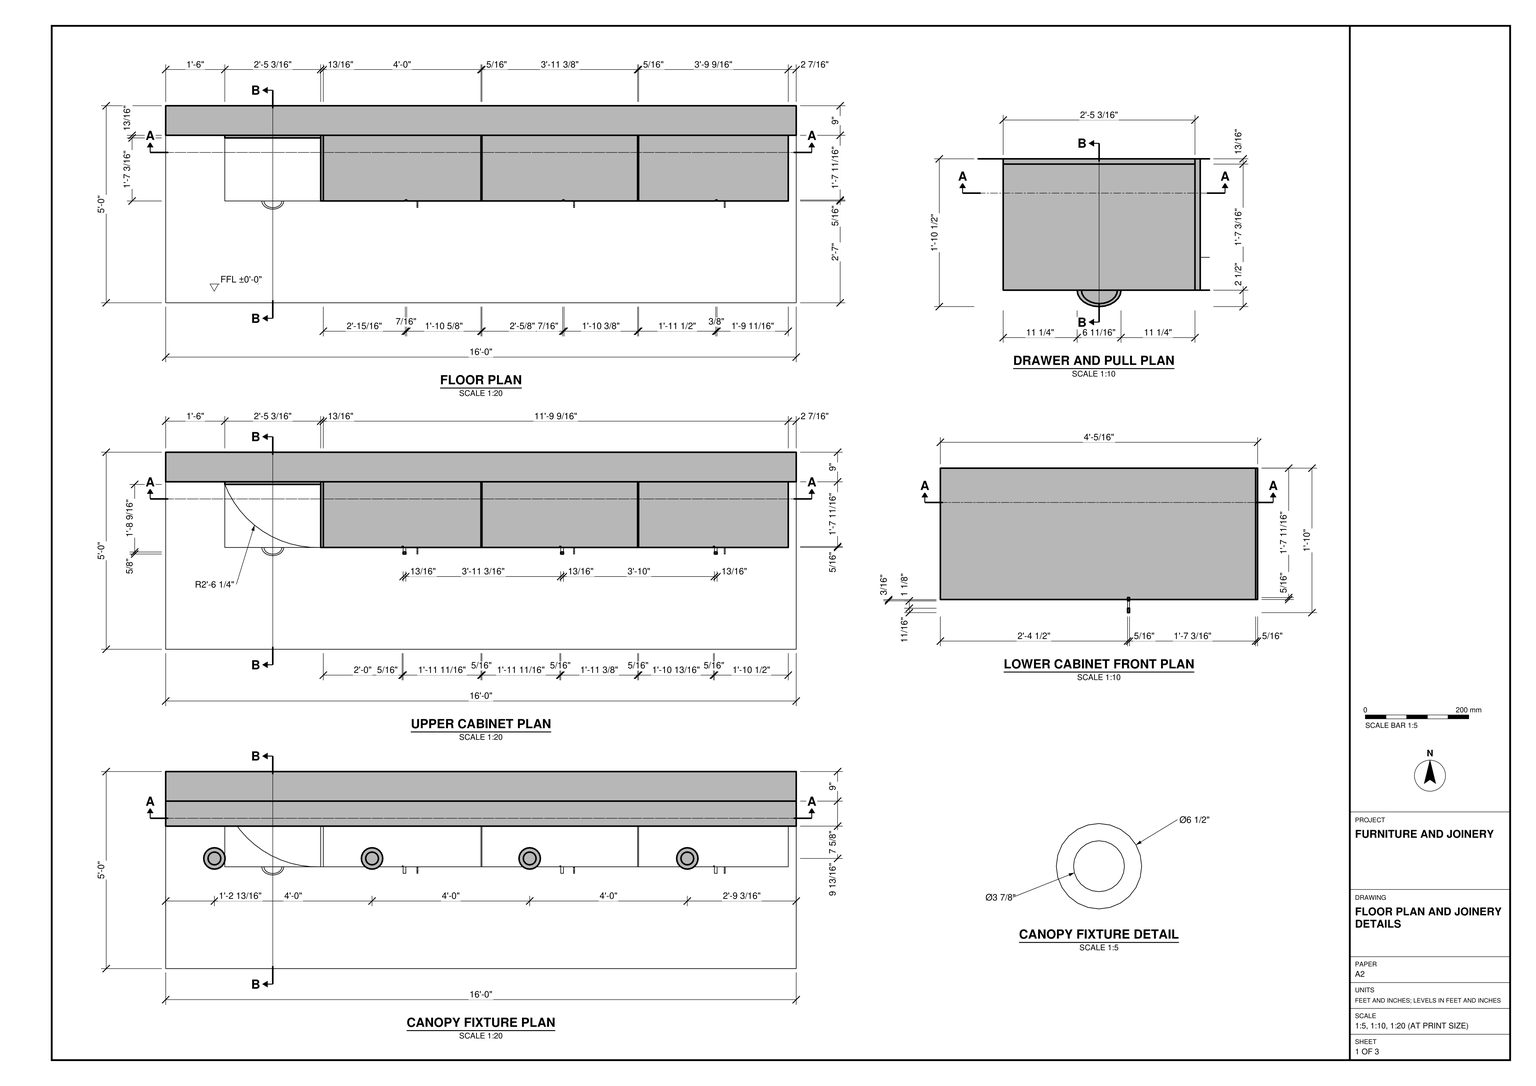
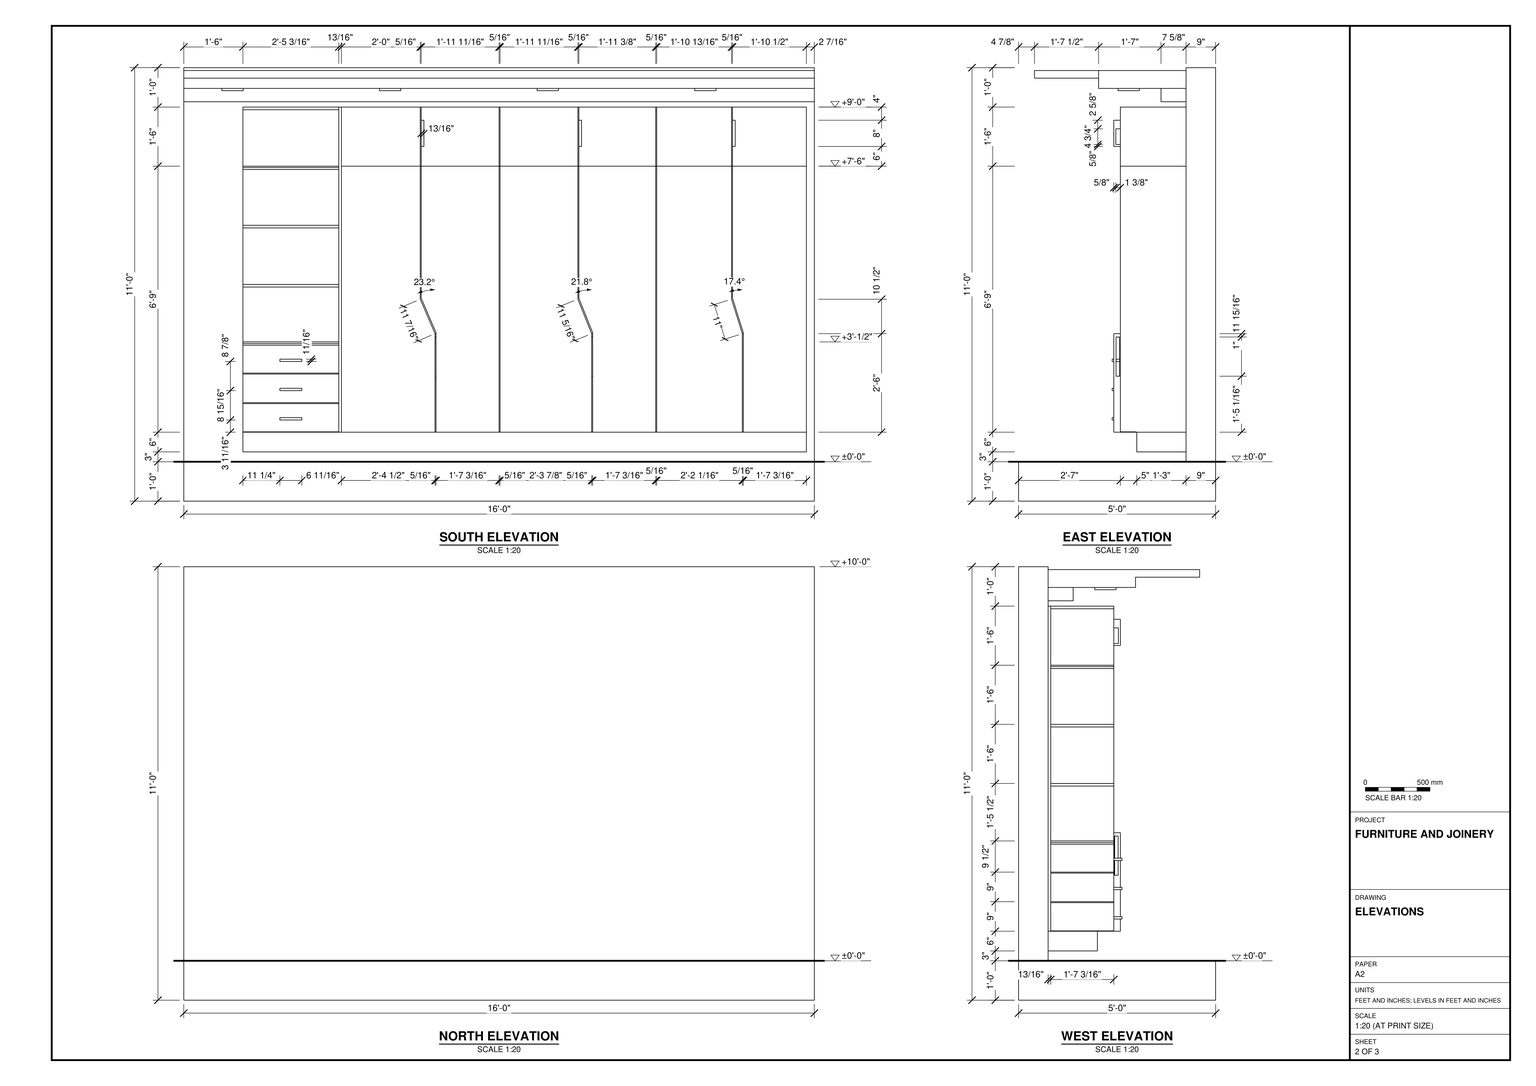
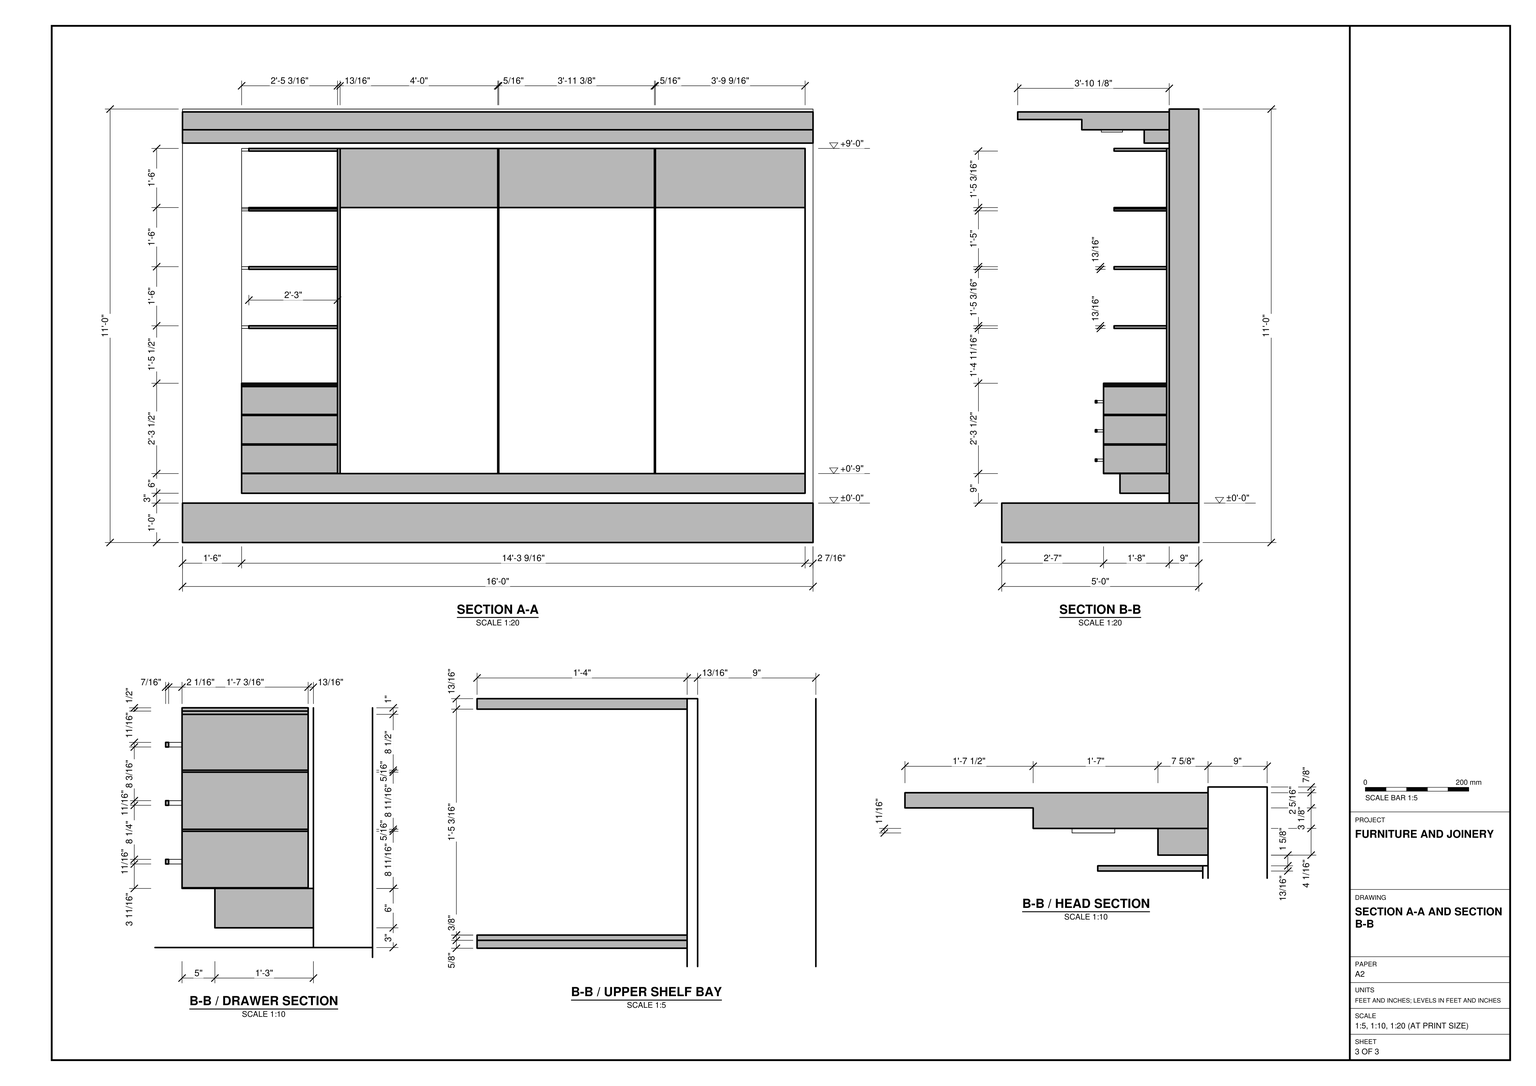
Build the storage wall in SketchUp from task_files/diagram_01.pdf. Work in feet and inches. The complete assembly is 16'-0" wide, 5'-0" deep and 11'-0" high. Use the top of the floor slab as the finished floor level, ±0'-0". The slab extends 1'-0" below this level, and the rear wall rises to +10'-0".

Use the south elevation to lay out the cabinet fronts. Leave 1'-6" between the left end of the wall and the narrow drawer and shelf bay. Model the three drawers with projecting pulls, the open shelves above them and the three wider cabinet bays to their right. Divide the wider bays into tall lower doors and a shorter row of upper doors. Follow the elevations for the door divisions and pull locations. Use the sections to set the shelf depths, panel thicknesses and recessed plinth rather than making the cabinet run a single solid block.

Above the cabinets, model the full-width projecting canopy with the stepped underside shown in the head section. Locate its fixtures from the canopy plan. Any decor or loose items shown may be represented by suitable library components. Keep the slab, rear wall, canopy and individual joinery pieces in separate groups or components, and use components for repeated parts. Save one SketchUp model as output_files/built_in_storage_wall_with_drawers_shelves_and_canopy.skp.

# SketchUp Ruby script. Lengths in inches.
U = 1.inch
M = Sketchup.active_model
def pt(a) = Geom::Point3d.new(a.map { |v| v * U })
def face(e, loops, mat)
  f = e.add_face(loops[0].map { |a| pt(a) })
  loops[1..].each { |l| e.add_face(l.map { |a| pt(a) }).erase! }
  f.material = f.back_material = mat if mat
  f
end
# faces: each face lists its corners as indices into pts; further lists are holes
def faces(e, pts, list, mat = nil) = list.each { |f| face(e, (f[0].is_a?(Array) ? f : [f]).map { |l| l.map { |i| pts[i] } }, mat) }
# xy, xz, yz: faces in a plane at the given z, y or x. An outline is a flat list of corners, or four numbers for a rectangle; further outlines are holes
def ring(l) = l.size == 4 ? [[l[0], l[1]], [l[2], l[1]], [l[2], l[3]], [l[0], l[3]]] : l.each_slice(2).to_a
def flat(e, list, mat, &to3) = list.each { |f| face(e, (f[0].is_a?(Array) ? f : [f]).map { |l| ring(l).map { |u, v| to3.(u, v) } }, mat) }
def xy(e, z, list, mat = nil) = flat(e, list, mat) { |x, y| [x, y, z] }
def xz(e, y, list, mat = nil) = flat(e, list, mat) { |x, z| [x, y, z] }
def yz(e, x, list, mat = nil) = flat(e, list, mat) { |y, z| [x, y, z] }
def lines(e, pts, list) = list.each { |a, b| e.add_line(pt(pts[a]), pt(pts[b])) }
# prism: a flat outline (further loops are holes) pulled along v
def prism(e, loops, v, mat = nil)
  f = face(e, loops, mat); d = Geom::Vector3d.new(v.map { |x| x * U })
  f.pushpull(f.normal.samedirection?(d) ? d.length : -d.length)
end
def box(e, o, s, mat = nil) = prism(e, [[o, [o[0] + s[0], o[1], o[2]], [o[0] + s[0], o[1] + s[1], o[2]], [o[0], o[1] + s[1], o[2]]]], [0, 0, s[2]], mat)
def at(x, y, z, deg = 0) = Geom::Transformation.translation(pt([x, y, z])) * Geom::Transformation.rotation(ORIGIN, Z_AXIS, deg.degrees)
def axes(o, x, y, z) = Geom::Transformation.new([*x, 0, *y, 0, *z, 0, *pt(o).to_a, 1])
def part(name) = M.definitions.add(name)
# library, detail: a bought-in or finely detailed component or shape, given as its bounding box
def library(name, o, s) = part(name).tap { |d| box(d.entities, o, s) }
def detail(e, o, s) = box(e.add_group.entities, o, s)
def put(e, d, t, mat = nil) = e.add_instance(d, t).tap { |i| i.material = mat if mat }
def group(e, t, mat = nil) = e.add_group.tap { |g| g.transformation = t; g.material = mat if mat }.entities
root = M.entities
M.materials.add("[Color D01]").color = [255, 242, 204]
M.materials.add("[Color M00]").color = [255, 255, 255]
M.materials.add("[Color M06]").color = [86, 86, 86]
M.materials.add("[Color M09]").color = [0, 0, 0]
M.materials.add("[Field Rectangle Tile]").color = [196, 189, 179]
M.materials.add("[Metal Corrugated Shiny]").color = [193, 193, 193]
M.materials.add("[Metal Rusted]").color = [184, 117, 91]
c1 = part("Group\#18")
prism(c1.entities,[[[0,1.91,0],[0.375,1.91,0],[0.43,1.5,0],[0.58,1.125,0],[0.83,0.8,0],[1.15,0.55,0],[1.53,0.4,0],[1.9375,0.34,0],[2.34,0.4,0],[2.72,0.55,0],[3.04,0.8,0],[3.29,1.125,0],[3.45,1.5,0],[3.5,1.91,0],[3.8125,1.91,0],[3.75,1.41,0],[3.56,0.95,0],[3.25,0.56,0],[2.86,0.26,0],[2.4,0.06,0],[1.91,0,0],[1.41,0.06,0],[0.95,0.26,0],[0.56,0.56,0],[0.26,0.95,0],[0.06,1.41,0]]],[0,0,0.5])
g1 = group(root,at(0,0,0))
xy(g1,0,[[0,0,192,60]])
xy(g1,12,[[0,0,192,60]],"[Field Rectangle Tile]")
xz(g1,0,[[0,0,192,12]])
xz(g1,60,[[0,0,192,12]])
yz(g1,0,[[0,0,60,12]])
yz(g1,192,[[0,0,60,12]])
g2 = group(root,at(0,51,12),"[Color D01]")
box(g2,[0,0,0],[192,9,120])
g3 = group(root,at(18,51,15),"[Color M06]")
g4 = group(g3,at(0,-15,0))
box(g4,[0,0,0],[171.58,15,6])
g5 = group(root,at(47.2,31,21),"[Color M06]")
box(g5,[0,0,0],[0.8,20,99])
g6 = group(root,at(48,31,21),"[Color M06]")
g7 = group(g6,at(0,0,81))
xy(g7,0,[[0,0,0,20,48,20,48,0,24.3,0,24.3,0.3,24,0.3,24,0],[48,0,48.3,20],[48.3,0,48.3,20,95.7,20,95.7,0,72.3,0,72.3,0.3,72,0.3,72,0],[95.7,0,96,20],[96,0,96,20,141.57,20,141.57,0,119.09,0,119.09,0.3,118.79,0.3,118.79,0]])
xy(g7,18,[[0,0,24,0,24,0.3,24.3,0.3,24.3,0,48,0,48,20,0,20],[48,0,48.3,20],[48.3,0,72,0,72,0.3,72.3,0.3,72.3,0,95.7,0,95.7,20,48.3,20],[95.7,0,96,20],[96,0,118.79,0,118.79,0.3,119.09,0.3,119.09,0,141.57,0,141.57,20,96,20]])
xz(g7,0,[[0,0,24,18],[24.3,0,48,18],[48,0,48.3,18],[48.3,0,72,18],[72.3,0,95.7,18],
  [95.7,0,96,18],[96,0,118.79,18],[119.09,0,141.57,18]])
xz(g7,0.3,[[24,0,24.3,18],[72,0,72.3,18],[118.79,0,119.09,18]])
xz(g7,20,[[0,0,48,18],[48,0,48.3,18],[48.3,0,95.7,18],[95.7,0,96,18],[96,0,141.57,18]])
yz(g7,0,[[0,0,20,18]])
yz(g7,24,[[0,0,0.3,18]])
yz(g7,24.3,[[0,0,0.3,18]])
yz(g7,48,[[0,0,20,18]])
yz(g7,48.3,[[0,0,20,18]])
yz(g7,72,[[0,0,0.3,18]])
yz(g7,72.3,[[0,0,0.3,18]])
yz(g7,95.7,[[0,0,20,18]])
yz(g7,96,[[0,0,20,18]])
yz(g7,118.79,[[0,0,0.3,18]])
yz(g7,119.09,[[0,0,0.3,18]])
yz(g7,141.57,[[0,0,20,18]])
g8 = group(g6,at(0,20,0))
g9 = group(g8,at(0,-20,0))
xy(g9,0,[[0,0,0,20,48,20,48,0,28.8,0,28.8,0.3,28.5,0.3,28.5,0],[48,0,48.3,20],[48.3,0,48.3,20,95.7,20,95.7,0,76.5,0,76.5,0.3,76.2,0.3,76.2,0],[95.7,0,96,20],[96,0,96,20,141.57,20,141.57,0,122.375,0,122.375,0.3,122.07,0.3,122.07,0]])
xy(g9,81,[[0,0,24,0,24,0.3,24.3,0.3,24.3,0,48,0,48,20,0,20],[48,0,48.3,20],[48.3,0,72,0,72,0.3,72.3,0.3,72.3,0,95.7,0,95.7,20,48.3,20],[95.7,0,96,20],[96,0,118.79,0,118.79,0.3,119.09,0.3,119.09,0,141.57,0,141.57,20,96,20]])
xz(g9,0,[[0,0,28.5,0,28.5,30,24,40.5,24,81,0,81],[28.8,0,48,0,48,81,24.3,81,24.3,40.8,28.8,30.3],[48,0,48.3,81],[48.3,0,76.2,0,76.2,30,72,40.5,72,81,48.3,81],[76.5,0,95.7,0,95.7,81,72.3,81,72.3,40.8,76.5,30.3],
  [95.7,0,96,81],[96,0,122.07,0,122.07,30,118.79,40.5,118.79,81,96,81],[122.375,0,141.57,0,141.57,81,119.09,81,119.09,40.8,122.375,30.3]])
xz(g9,0.3,[[28.5,0,28.8,0,28.8,30.3,24.3,40.8,24.3,81,24,81,24,40.5,28.5,30],[76.2,0,76.5,0,76.5,30.3,72.3,40.8,72.3,81,72,81,72,40.5,76.2,30],[122.07,0,122.375,0,122.375,30.3,119.09,40.8,119.09,81,118.79,81,118.79,40.5,122.07,30]])
xz(g9,20,[[0,0,48,81],[48,0,48.3,81],[48.3,0,95.7,81],[95.7,0,96,81],[96,0,141.57,81]])
yz(g9,0,[[0,0,20,81]])
yz(g9,24,[[0,40.5,0.3,81]])
yz(g9,24.3,[[0,40.8,0.3,81]])
yz(g9,28.5,[[0,0,0.3,30]])
yz(g9,28.8,[[0,0,0.3,30.3]])
yz(g9,48,[[0,0,20,81]])
yz(g9,48.3,[[0,0,20,81]])
yz(g9,72,[[0,40.5,0.3,81]])
yz(g9,72.3,[[0,40.8,0.3,81]])
yz(g9,76.2,[[0,0,0.3,30]])
yz(g9,76.5,[[0,0,0.3,30.3]])
yz(g9,95.7,[[0,0,20,81]])
yz(g9,96,[[0,0,20,81]])
yz(g9,118.79,[[0,40.5,0.3,81]])
yz(g9,119.09,[[0,40.8,0.3,81]])
yz(g9,122.07,[[0,0,0.3,30]])
yz(g9,122.375,[[0,0,0.3,30.3]])
yz(g9,141.57,[[0,0,20,81]])
p = [[24,0,40.5],[28.5,0,30],[28.5,0.3,30],[24,0.3,40.5],[72,0,40.5],[76.2,0,30],
  [76.2,0.3,30],[72,0.3,40.5],[118.79,0,40.5],[122.07,0,30],[122.07,0.3,30],[118.79,0.3,40.5],
  [28.8,0,30.3],[24.3,0,40.8],[24.3,0.3,40.8],[28.8,0.3,30.3],[76.5,0,30.3],[72.3,0,40.8],
  [72.3,0.3,40.8],[76.5,0.3,30.3],[122.375,0,30.3],[119.09,0,40.8],[119.09,0.3,40.8],[122.375,0.3,30.3]]
faces(g9,p,[[0,1,2,3],[4,5,6,7],[8,9,10,11],[12,13,14,15],[16,17,18,19],[20,21,22,23]])
g10 = group(root,at(76.5,29,21),"[Color M09]")
prism(g10,[[[0,2,30],[0,2,0],[0,0,0],[0,0,30]],[[0,1.8,28.99],[0,0.68,28.99],[0,0.68,17.05],[0,1.8,17.05]]],[0.3,0,0])
g11 = group(root,at(124.2,29,21),"[Color M09]")
prism(g11,[[[0,2,30],[0,2,0],[0,0,0],[0,0,30]],[[0,1.8,28.99],[0,0.68,28.99],[0,0.68,17.05],[0,1.8,17.05]]],[0.3,0,0])
g12 = group(root,at(170.08,29,21),"[Color M09]")
prism(g12,[[[0,2,30],[0,2,0],[0,0,0],[0,0,30]],[[0,1.74,28.99],[0,0.68,28.99],[0,0.68,17.05],[0,1.74,17.05]]],[0.3,0,0])
g13 = group(root,at(18,50.2,21),"[Color M06]")
box(g13,[0,0,0],[29.2,0.8,99])
g14 = group(root,at(18,31,119.7),"[Color M06]")
prism(g14,[[[29.2,19.2,-0.5],[29.2,0,-0.5],[26.1,0.05,-0.5],[23.01,0.42,-0.5],[19.99,1.1,-0.5],[17.05,2.1,-0.5],[14.22,3.38,-0.5],[11.54,4.95,-0.5],[9.04,6.79,-0.5],[6.74,8.87,-0.5],[4.67,11.18,-0.5],[2.84,13.6875,-0.5],[1.28,16.37,-0.5],[0,19.2,-0.5]]],[0,0,0.8])
g15 = group(root,at(18,31,101.6),"[Color M06]")
prism(g15,[[[29.2,19.2,0],[29.2,0,0],[26.1,0.05,0],[23.01,0.42,0],[19.99,1.1,0],[17.05,2.1,0],[14.22,3.38,0],[11.54,4.95,0],[9.04,6.79,0],[6.74,8.87,0],[4.67,11.18,0],[2.84,13.6875,0],[1.28,16.37,0],[0,19.2,0]]],[0,0,0.4])
g16 = group(root,at(18,31,83.7),"[Color M06]")
prism(g16,[[[29.2,19.2,-0.5],[29.2,0,-0.5],[26.1,0.05,-0.5],[23.01,0.42,-0.5],[19.99,1.1,-0.5],[17.05,2.1,-0.5],[14.22,3.38,-0.5],[11.54,4.95,-0.5],[9.04,6.79,-0.5],[6.74,8.87,-0.5],[4.67,11.18,-0.5],[2.84,13.6875,-0.5],[1.28,16.37,-0.5],[0,19.2,-0.5]]],[0,0,0.8])
g17 = group(root,at(18,31,65.7),"[Color M06]")
prism(g17,[[[29.2,19.2,-0.5],[29.2,0,-0.5],[26.1,0.05,-0.5],[23.01,0.42,-0.5],[19.99,1.1,-0.5],[17.05,2.1,-0.5],[14.22,3.38,-0.5],[11.54,4.95,-0.5],[9.04,6.79,-0.5],[6.74,8.87,-0.5],[4.67,11.18,-0.5],[2.84,13.6875,-0.5],[1.28,16.37,-0.5],[0,19.2,-0.5]]],[0,0,0.8])
g18 = group(root,at(18,31,101.3),"[Color M06]")
prism(g18,[[[29.2,19.2,-0.3],[29.2,0,-0.3],[26.1,0.05,-0.3],[23.01,0.42,-0.3],[19.99,1.1,-0.3],[17.05,2.1,-0.3],[14.22,3.38,-0.3],[11.54,4.95,-0.3],[9.04,6.79,-0.3],[6.74,8.87,-0.3],[4.67,11.18,-0.3],[2.84,13.6875,-0.3],[1.28,16.37,-0.3],[0,19.2,-0.3]]],[0,0,0.6])
g19 = group(root,at(18,31,21),"[Color M06]")
xy(g19,0,[[0,0,29.2,19.2]])
xy(g19,0.1,[[0,0,29.2,19.2]])
xy(g19,8.7,[[0,0,29.2,19.2]])
xy(g19,9,[[0,0,29.2,19.2]])
xy(g19,17.7,[[0,0,29.2,19.2]])
xy(g19,18,[[0,0,29.2,19.2]])
xy(g19,26.5,[[0,0,29.2,19.2]])
xy(g19,27,[[0,0,29.2,19.2]])
xy(g19,27.5,[[0,0,29.2,19.2]])
xz(g19,0,[[0,0,29.2,0.1],[0,0.1,29.2,8.7],[0,8.7,29.2,9],[0,9,29.2,17.7],[0,17.7,29.2,18],
  [0,18,29.2,26.5],[0,26.5,29.2,27],[0,27,29.2,27.5]])
xz(g19,19.2,[[0,0,29.2,0.1],[0,0.1,29.2,8.7],[0,8.7,29.2,9],[0,9,29.2,17.7],[0,17.7,29.2,18],
  [0,18,29.2,26.5],[0,26.5,29.2,27],[0,27,29.2,27.5]])
yz(g19,0,[[0,0,19.2,0.1],[0,0.1,19.2,8.7],[0,8.7,19.2,9],[0,9,19.2,17.7],[0,17.7,19.2,18],
  [0,18,19.2,26.5],[0,26.5,19.2,27],[0,27,19.2,27.5]])
yz(g19,29.2,[[0,0,19.2,0.1],[0,0.1,19.2,8.7],[0,8.7,19.2,9],[0,9,19.2,17.7],[0,17.7,19.2,18],
  [0,18,19.2,26.5],[0,26.5,19.2,27],[0,27,19.2,27.5]])
put(root,c1,axes([29.26,28.5,42.53],[1.75218,0,0],[0,1.31,0],[0,0,1.41]),"[Color M09]")
put(root,c1,axes([29.26,28.5,33.66],[1.75218,0,0],[0,1.31,0],[0,0,1.41]),"[Color M09]")
put(root,c1,axes([29.26,28.5,24.72],[1.75218,0,0],[0,1.31,0],[0,0,1.41]),"[Color M09]")
g20 = group(root,at(72.3,29,108),"[Color M09]")
prism(g20,[[[0.82,2,5.38],[0.82,2,8],[0.82,0,8],[0.82,0,0],[0.82,2,0],[0.82,2,0.62],[0.82,0.62,0.62],[0.82,0.62,5.38]]],[-0.82,0,0])
g21 = group(root,at(120.3,29,108),"[Color M09]")
prism(g21,[[[0.82,2,5.38],[0.82,2,8],[0.82,0,8],[0.82,0,0],[0.82,2,0],[0.82,2,0.62],[0.82,0.62,0.62],[0.82,0.62,5.38]]],[-0.82,0,0])
g22 = group(root,at(167.09,29,108),"[Color M09]")
prism(g22,[[[0.82,2,5.38],[0.82,2,8],[0.82,0,8],[0.82,0,0],[0.82,2,0],[0.82,2,0.62],[0.82,0.62,0.62],[0.82,0.62,5.38]]],[-0.82,0,0])
g23 = group(root,at(0,46,122),"[Color D01]")
xy(g23,-0.375,[[0,-2.625,192,5]])
xy(g23,3.6875,[[0,-2.625,192,5]],"[Color D01]")
xz(g23,-2.625,[[0,-0.375,192,3.6875]],"[Color D01]")
xz(g23,5,[[0,-0.375,192,3.6875]])
yz(g23,0,[[-2.625,-0.375,5,3.6875]])
yz(g23,192,[[-2.625,-0.375,5,3.6875]])
g24 = group(root,at(0,4.85,125.6875),"[Color M00]")
xy(g24,0,[[0,19.52,192,46.15]])
xy(g24,3.125,[[0,0,192,19.52]])
xy(g24,5.4375,[[0,0,192,46.15]])
xz(g24,0,[[0,3.125,192,5.4375]])
xz(g24,19.52,[[0,0,192,3.125]])
xz(g24,46.15,[[0,0,192,5.4375]])
yz(g24,0,[[19.52,0,19.52,3.125,0,3.125,0,5.4375,46.15,5.4375,46.15,0]])
yz(g24,192,[[19.52,0,46.15,5.4375],[0,3.125,19.52,5.4375]])
g25 = group(root,at(11.59,30.3,125),"[Metal Rusted]")
xy(g25,0,[[[3.25,0,2.41,0.11,1.625,0.44,0.95,0.95,0.44,1.625,0.11,2.41,0,3.25,0.11,4.09,0.44,4.875,0.95,5.55,1.625,6.06,2.41,6.39,3.25,6.5,4.09,6.39,4.875,6.06,5.55,5.55,6.06,4.875,6.39,4.09,6.5,3.25,6.39,2.41,6.06,1.625,5.55,0.95,4.875,0.44,4.09,0.11],[3.25,1.3125,3.75,1.38,4.22,1.57,4.62,1.88,4.93,2.28,5.12,2.75,5.1875,3.25,5.12,3.75,4.93,4.22,4.62,4.62,4.22,4.93,3.75,5.12,3.25,5.1875,2.75,5.12,2.28,4.93,1.88,4.62,1.57,4.22,1.38,3.75,1.3125,3.25,1.38,2.75,1.57,2.28,1.88,1.88,2.28,1.57,2.75,1.38]]])
xy(g25,0.4375,[[3.25,1.3125,3.75,1.38,4.22,1.57,4.62,1.88,4.93,2.28,5.12,2.75,5.1875,3.25,5.12,3.75,4.93,4.22,4.62,4.62,4.22,4.93,3.75,5.12,3.25,5.1875,2.75,5.12,2.28,4.93,1.88,4.62,1.57,4.22,1.38,3.75,1.3125,3.25,1.38,2.75,1.57,2.28,1.88,1.88,2.28,1.57,2.75,1.38]],"[Metal Corrugated Shiny]")
xy(g25,0.6875,[[[3.25,0,4.09,0.11,4.875,0.44,5.55,0.95,6.06,1.625,6.39,2.41,6.5,3.25,6.39,4.09,6.06,4.875,5.55,5.55,4.875,6.06,4.09,6.39,3.25,6.5,2.41,6.39,1.625,6.06,0.95,5.55,0.44,4.875,0.11,4.09,0,3.25,0.11,2.41,0.44,1.625,0.95,0.95,1.625,0.44,2.41,0.11],[3.25,1.3125,2.75,1.38,2.28,1.57,1.88,1.88,1.57,2.28,1.38,2.75,1.3125,3.25,1.38,3.75,1.57,4.22,1.88,4.62,2.28,4.93,2.75,5.12,3.25,5.1875,3.75,5.12,4.22,4.93,4.62,4.62,4.93,4.22,5.12,3.75,5.1875,3.25,5.12,2.75,4.93,2.28,4.62,1.88,4.22,1.57,3.75,1.38]]])
p = [[3.25,0,0.6875],[2.41,0.11,0.6875],[2.41,0.11,0],[3.25,0,0],[4.09,0.11,0.6875],[4.09,0.11,0],
  [1.625,0.44,0.6875],[1.625,0.44,0],[4.875,0.44,0.6875],[4.875,0.44,0],[0.95,0.95,0.6875],[0.95,0.95,0],
  [5.55,0.95,0.6875],[5.55,0.95,0],[0.44,1.625,0.6875],[0.44,1.625,0],[6.06,1.625,0.6875],[6.06,1.625,0],
  [2.75,1.38,0],[2.75,1.38,0.4375],[3.25,1.3125,0.4375],[3.25,1.3125,0],[3.75,1.38,0.4375],[3.75,1.38,0],
  [2.28,1.57,0],[2.28,1.57,0.4375],[4.22,1.57,0.4375],[4.22,1.57,0],[0.11,2.41,0.6875],[0.11,2.41,0],
  [1.88,1.88,0],[1.88,1.88,0.4375],[4.62,1.88,0.4375],[4.62,1.88,0],[6.39,2.41,0.6875],[6.39,2.41,0],
  [1.57,2.28,0],[1.57,2.28,0.4375],[4.93,2.28,0.4375],[4.93,2.28,0],[1.38,2.75,0],[1.38,2.75,0.4375],
  [5.12,2.75,0.4375],[5.12,2.75,0],[0,3.25,0.6875],[0,3.25,0],[6.5,3.25,0.6875],[6.5,3.25,0],
  [1.3125,3.25,0],[1.3125,3.25,0.4375],[5.1875,3.25,0.4375],[5.1875,3.25,0],[0.11,4.09,0.6875],[0.11,4.09,0],
  [1.38,3.75,0],[1.38,3.75,0.4375],[5.12,3.75,0.4375],[5.12,3.75,0],[6.39,4.09,0.6875],[6.39,4.09,0],
  [1.57,4.22,0],[1.57,4.22,0.4375],[4.93,4.22,0.4375],[4.93,4.22,0],[0.44,4.875,0.6875],[0.44,4.875,0],
  [6.06,4.875,0.6875],[6.06,4.875,0],[1.88,4.62,0],[1.88,4.62,0.4375],[4.62,4.62,0.4375],[4.62,4.62,0],
  [2.28,4.93,0],[2.28,4.93,0.4375],[4.22,4.93,0.4375],[4.22,4.93,0],[0.95,5.55,0.6875],[0.95,5.55,0],
  [2.75,5.12,0],[2.75,5.12,0.4375],[3.75,5.12,0.4375],[3.75,5.12,0],[5.55,5.55,0.6875],[5.55,5.55,0],
  [3.25,5.1875,0],[3.25,5.1875,0.4375],[1.625,6.06,0.6875],[1.625,6.06,0],[4.875,6.06,0.6875],[4.875,6.06,0],
  [2.41,6.39,0.6875],[2.41,6.39,0],[4.09,6.39,0.6875],[4.09,6.39,0],[3.25,6.5,0.6875],[3.25,6.5,0],
  [2.75,1.38,0.6875],[3.25,1.3125,0.6875],[3.75,1.38,0.6875],[2.28,1.57,0.6875],[4.22,1.57,0.6875],[1.88,1.88,0.6875],
  [4.62,1.88,0.6875],[1.57,2.28,0.6875],[4.93,2.28,0.6875],[1.38,2.75,0.6875],[5.12,2.75,0.6875],[1.3125,3.25,0.6875],
  [5.1875,3.25,0.6875],[1.38,3.75,0.6875],[5.12,3.75,0.6875],[1.57,4.22,0.6875],[4.93,4.22,0.6875],[1.88,4.62,0.6875],
  [4.62,4.62,0.6875],[2.28,4.93,0.6875],[4.22,4.93,0.6875],[2.75,5.12,0.6875],[3.75,5.12,0.6875],[3.25,5.1875,0.6875]]
faces(g25,p,[[0,1,2,3],[4,0,3,5],[1,6,7,2],[8,4,5,9],[6,10,11,7],[12,8,9,13],[10,14,15,11],[16,12,13,17],
  [14,28,29,15],[34,16,17,35],[28,44,45,29],[46,34,35,47],[44,52,53,45],[58,46,47,59],[52,64,65,53],[66,58,59,67],
  [64,76,77,65],[82,66,67,83],[76,86,87,77],[88,82,83,89],[86,90,91,87],[92,88,89,93],[90,94,95,91],[94,92,93,95],
  [96,97,20,19],[97,98,22,20],[99,96,19,25],[98,100,26,22],[101,99,25,31],[100,102,32,26],[103,101,31,37],[102,104,38,32],
  [105,103,37,41],[104,106,42,38],[107,105,41,49],[106,108,50,42],[109,107,49,55],[108,110,56,50],[111,109,55,61],[110,112,62,56],
  [113,111,61,69],[112,114,70,62],[115,113,69,73],[114,116,74,70],[117,115,73,79],[116,118,80,74],[119,117,79,85],[118,119,85,80]])
faces(g25,p,[[18,19,20,21],[21,20,22,23],[24,25,19,18],[23,22,26,27],[30,31,25,24],[27,26,32,33],[36,37,31,30],[33,32,38,39],
  [40,41,37,36],[39,38,42,43],[48,49,41,40],[43,42,50,51],[54,55,49,48],[51,50,56,57],[60,61,55,54],[57,56,62,63],
  [68,69,61,60],[63,62,70,71],[72,73,69,68],[71,70,74,75],[78,79,73,72],[75,74,80,81],[84,85,79,78],[81,80,85,84]],"[Metal Corrugated Shiny]")
g26 = group(root,at(59.59,30.3,125),"[Metal Rusted]")
xy(g26,0,[[[3.25,0,2.41,0.11,1.625,0.44,0.95,0.95,0.44,1.625,0.11,2.41,0,3.25,0.11,4.09,0.44,4.875,0.95,5.55,1.625,6.06,2.41,6.39,3.25,6.5,4.09,6.39,4.875,6.06,5.55,5.55,6.06,4.875,6.39,4.09,6.5,3.25,6.39,2.41,6.06,1.625,5.55,0.95,4.875,0.44,4.09,0.11],[3.25,1.3125,3.75,1.38,4.22,1.57,4.62,1.88,4.93,2.28,5.12,2.75,5.1875,3.25,5.12,3.75,4.93,4.22,4.62,4.62,4.22,4.93,3.75,5.12,3.25,5.1875,2.75,5.12,2.28,4.93,1.88,4.62,1.57,4.22,1.38,3.75,1.3125,3.25,1.38,2.75,1.57,2.28,1.88,1.88,2.28,1.57,2.75,1.38]]],"[Metal Corrugated Shiny]")
xy(g26,0.4375,[[3.25,1.3125,3.75,1.38,4.22,1.57,4.62,1.88,4.93,2.28,5.12,2.75,5.1875,3.25,5.12,3.75,4.93,4.22,4.62,4.62,4.22,4.93,3.75,5.12,3.25,5.1875,2.75,5.12,2.28,4.93,1.88,4.62,1.57,4.22,1.38,3.75,1.3125,3.25,1.38,2.75,1.57,2.28,1.88,1.88,2.28,1.57,2.75,1.38]],"[Metal Corrugated Shiny]")
xy(g26,0.6875,[[[3.25,0,4.09,0.11,4.875,0.44,5.55,0.95,6.06,1.625,6.39,2.41,6.5,3.25,6.39,4.09,6.06,4.875,5.55,5.55,4.875,6.06,4.09,6.39,3.25,6.5,2.41,6.39,1.625,6.06,0.95,5.55,0.44,4.875,0.11,4.09,0,3.25,0.11,2.41,0.44,1.625,0.95,0.95,1.625,0.44,2.41,0.11],[3.25,1.3125,2.75,1.38,2.28,1.57,1.88,1.88,1.57,2.28,1.38,2.75,1.3125,3.25,1.38,3.75,1.57,4.22,1.88,4.62,2.28,4.93,2.75,5.12,3.25,5.1875,3.75,5.12,4.22,4.93,4.62,4.62,4.93,4.22,5.12,3.75,5.1875,3.25,5.12,2.75,4.93,2.28,4.62,1.88,4.22,1.57,3.75,1.38]]],"[Metal Corrugated Shiny]")
p = [[3.25,0,0.6875],[2.41,0.11,0.6875],[2.41,0.11,0],[3.25,0,0],[4.09,0.11,0.6875],[4.09,0.11,0],
  [1.625,0.44,0.6875],[1.625,0.44,0],[4.875,0.44,0.6875],[4.875,0.44,0],[0.95,0.95,0.6875],[0.95,0.95,0],
  [5.55,0.95,0.6875],[5.55,0.95,0],[0.44,1.625,0.6875],[0.44,1.625,0],[6.06,1.625,0.6875],[6.06,1.625,0],
  [2.75,1.38,0],[2.75,1.38,0.4375],[3.25,1.3125,0.4375],[3.25,1.3125,0],[3.75,1.38,0.4375],[3.75,1.38,0],
  [2.28,1.57,0],[2.28,1.57,0.4375],[4.22,1.57,0.4375],[4.22,1.57,0],[0.11,2.41,0.6875],[0.11,2.41,0],
  [1.88,1.88,0],[1.88,1.88,0.4375],[4.62,1.88,0.4375],[4.62,1.88,0],[6.39,2.41,0.6875],[6.39,2.41,0],
  [1.57,2.28,0],[1.57,2.28,0.4375],[4.93,2.28,0.4375],[4.93,2.28,0],[1.38,2.75,0],[1.38,2.75,0.4375],
  [5.12,2.75,0.4375],[5.12,2.75,0],[0,3.25,0.6875],[0,3.25,0],[6.5,3.25,0.6875],[6.5,3.25,0],
  [1.3125,3.25,0],[1.3125,3.25,0.4375],[5.1875,3.25,0.4375],[5.1875,3.25,0],[0.11,4.09,0.6875],[0.11,4.09,0],
  [1.38,3.75,0],[1.38,3.75,0.4375],[5.12,3.75,0.4375],[5.12,3.75,0],[6.39,4.09,0.6875],[6.39,4.09,0],
  [1.57,4.22,0],[1.57,4.22,0.4375],[4.93,4.22,0.4375],[4.93,4.22,0],[0.44,4.875,0.6875],[0.44,4.875,0],
  [6.06,4.875,0.6875],[6.06,4.875,0],[1.88,4.62,0],[1.88,4.62,0.4375],[4.62,4.62,0.4375],[4.62,4.62,0],
  [2.28,4.93,0],[2.28,4.93,0.4375],[4.22,4.93,0.4375],[4.22,4.93,0],[0.95,5.55,0.6875],[0.95,5.55,0],
  [2.75,5.12,0],[2.75,5.12,0.4375],[3.75,5.12,0.4375],[3.75,5.12,0],[5.55,5.55,0.6875],[5.55,5.55,0],
  [3.25,5.1875,0],[3.25,5.1875,0.4375],[1.625,6.06,0.6875],[1.625,6.06,0],[4.875,6.06,0.6875],[4.875,6.06,0],
  [2.41,6.39,0.6875],[2.41,6.39,0],[4.09,6.39,0.6875],[4.09,6.39,0],[3.25,6.5,0.6875],[3.25,6.5,0],
  [2.75,1.38,0.6875],[3.25,1.3125,0.6875],[3.75,1.38,0.6875],[2.28,1.57,0.6875],[4.22,1.57,0.6875],[1.88,1.88,0.6875],
  [4.62,1.88,0.6875],[1.57,2.28,0.6875],[4.93,2.28,0.6875],[1.38,2.75,0.6875],[5.12,2.75,0.6875],[1.3125,3.25,0.6875],
  [5.1875,3.25,0.6875],[1.38,3.75,0.6875],[5.12,3.75,0.6875],[1.57,4.22,0.6875],[4.93,4.22,0.6875],[1.88,4.62,0.6875],
  [4.62,4.62,0.6875],[2.28,4.93,0.6875],[4.22,4.93,0.6875],[2.75,5.12,0.6875],[3.75,5.12,0.6875],[3.25,5.1875,0.6875]]
faces(g26,p,[[0,1,2,3],[4,0,3,5],[1,6,7,2],[8,4,5,9],[6,10,11,7],[12,8,9,13],[10,14,15,11],[16,12,13,17],
  [18,19,20,21],[21,20,22,23],[24,25,19,18],[23,22,26,27],[14,28,29,15],[30,31,25,24],[27,26,32,33],[34,16,17,35],
  [36,37,31,30],[33,32,38,39],[40,41,37,36],[39,38,42,43],[28,44,45,29],[46,34,35,47],[48,49,41,40],[43,42,50,51],
  [44,52,53,45],[54,55,49,48],[51,50,56,57],[58,46,47,59],[60,61,55,54],[57,56,62,63],[52,64,65,53],[66,58,59,67],
  [68,69,61,60],[63,62,70,71],[72,73,69,68],[71,70,74,75],[64,76,77,65],[78,79,73,72],[75,74,80,81],[82,66,67,83],
  [84,85,79,78],[81,80,85,84],[76,86,87,77],[88,82,83,89],[86,90,91,87],[92,88,89,93],[90,94,95,91],[94,92,93,95],
  [96,97,20,19],[97,98,22,20],[99,96,19,25],[98,100,26,22],[101,99,25,31],[100,102,32,26],[103,101,31,37],[102,104,38,32],
  [105,103,37,41],[104,106,42,38],[107,105,41,49],[106,108,50,42],[109,107,49,55],[108,110,56,50],[111,109,55,61],[110,112,62,56],
  [113,111,61,69],[112,114,70,62],[115,113,69,73],[114,116,74,70],[117,115,73,79],[116,118,80,74],[119,117,79,85],[118,119,85,80]],"[Metal Corrugated Shiny]")
g27 = group(root,at(107.59,30.3,125),"[Metal Rusted]")
xy(g27,0,[[[3.25,0,2.41,0.11,1.625,0.44,0.95,0.95,0.44,1.625,0.11,2.41,0,3.25,0.11,4.09,0.44,4.875,0.95,5.55,1.625,6.06,2.41,6.39,3.25,6.5,4.09,6.39,4.875,6.06,5.55,5.55,6.06,4.875,6.39,4.09,6.5,3.25,6.39,2.41,6.06,1.625,5.55,0.95,4.875,0.44,4.09,0.11],[3.25,1.3125,3.75,1.38,4.22,1.57,4.62,1.88,4.93,2.28,5.12,2.75,5.1875,3.25,5.12,3.75,4.93,4.22,4.62,4.62,4.22,4.93,3.75,5.12,3.25,5.1875,2.75,5.12,2.28,4.93,1.88,4.62,1.57,4.22,1.38,3.75,1.3125,3.25,1.38,2.75,1.57,2.28,1.88,1.88,2.28,1.57,2.75,1.38]]])
xy(g27,0.4375,[[3.25,1.3125,3.75,1.38,4.22,1.57,4.62,1.88,4.93,2.28,5.12,2.75,5.1875,3.25,5.12,3.75,4.93,4.22,4.62,4.62,4.22,4.93,3.75,5.12,3.25,5.1875,2.75,5.12,2.28,4.93,1.88,4.62,1.57,4.22,1.38,3.75,1.3125,3.25,1.38,2.75,1.57,2.28,1.88,1.88,2.28,1.57,2.75,1.38]],"[Metal Corrugated Shiny]")
xy(g27,0.6875,[[[3.25,0,4.09,0.11,4.875,0.44,5.55,0.95,6.06,1.625,6.39,2.41,6.5,3.25,6.39,4.09,6.06,4.875,5.55,5.55,4.875,6.06,4.09,6.39,3.25,6.5,2.41,6.39,1.625,6.06,0.95,5.55,0.44,4.875,0.11,4.09,0,3.25,0.11,2.41,0.44,1.625,0.95,0.95,1.625,0.44,2.41,0.11],[3.25,1.3125,2.75,1.38,2.28,1.57,1.88,1.88,1.57,2.28,1.38,2.75,1.3125,3.25,1.38,3.75,1.57,4.22,1.88,4.62,2.28,4.93,2.75,5.12,3.25,5.1875,3.75,5.12,4.22,4.93,4.62,4.62,4.93,4.22,5.12,3.75,5.1875,3.25,5.12,2.75,4.93,2.28,4.62,1.88,4.22,1.57,3.75,1.38]]])
p = [[3.25,0,0.6875],[2.41,0.11,0.6875],[2.41,0.11,0],[3.25,0,0],[4.09,0.11,0.6875],[4.09,0.11,0],
  [1.625,0.44,0.6875],[1.625,0.44,0],[4.875,0.44,0.6875],[4.875,0.44,0],[0.95,0.95,0.6875],[0.95,0.95,0],
  [5.55,0.95,0.6875],[5.55,0.95,0],[0.44,1.625,0.6875],[0.44,1.625,0],[6.06,1.625,0.6875],[6.06,1.625,0],
  [2.75,1.38,0],[2.75,1.38,0.4375],[3.25,1.3125,0.4375],[3.25,1.3125,0],[3.75,1.38,0.4375],[3.75,1.38,0],
  [2.28,1.57,0],[2.28,1.57,0.4375],[4.22,1.57,0.4375],[4.22,1.57,0],[0.11,2.41,0.6875],[0.11,2.41,0],
  [1.88,1.88,0],[1.88,1.88,0.4375],[4.62,1.88,0.4375],[4.62,1.88,0],[6.39,2.41,0.6875],[6.39,2.41,0],
  [1.57,2.28,0],[1.57,2.28,0.4375],[4.93,2.28,0.4375],[4.93,2.28,0],[1.38,2.75,0],[1.38,2.75,0.4375],
  [5.12,2.75,0.4375],[5.12,2.75,0],[0,3.25,0.6875],[0,3.25,0],[6.5,3.25,0.6875],[6.5,3.25,0],
  [1.3125,3.25,0],[1.3125,3.25,0.4375],[5.1875,3.25,0.4375],[5.1875,3.25,0],[0.11,4.09,0.6875],[0.11,4.09,0],
  [1.38,3.75,0],[1.38,3.75,0.4375],[5.12,3.75,0.4375],[5.12,3.75,0],[6.39,4.09,0.6875],[6.39,4.09,0],
  [1.57,4.22,0],[1.57,4.22,0.4375],[4.93,4.22,0.4375],[4.93,4.22,0],[0.44,4.875,0.6875],[0.44,4.875,0],
  [6.06,4.875,0.6875],[6.06,4.875,0],[1.88,4.62,0],[1.88,4.62,0.4375],[4.62,4.62,0.4375],[4.62,4.62,0],
  [2.28,4.93,0],[2.28,4.93,0.4375],[4.22,4.93,0.4375],[4.22,4.93,0],[0.95,5.55,0.6875],[0.95,5.55,0],
  [2.75,5.12,0],[2.75,5.12,0.4375],[3.75,5.12,0.4375],[3.75,5.12,0],[5.55,5.55,0.6875],[5.55,5.55,0],
  [3.25,5.1875,0],[3.25,5.1875,0.4375],[1.625,6.06,0.6875],[1.625,6.06,0],[4.875,6.06,0.6875],[4.875,6.06,0],
  [2.41,6.39,0.6875],[2.41,6.39,0],[4.09,6.39,0.6875],[4.09,6.39,0],[3.25,6.5,0.6875],[3.25,6.5,0],
  [2.75,1.38,0.6875],[3.25,1.3125,0.6875],[3.75,1.38,0.6875],[2.28,1.57,0.6875],[4.22,1.57,0.6875],[1.88,1.88,0.6875],
  [4.62,1.88,0.6875],[1.57,2.28,0.6875],[4.93,2.28,0.6875],[1.38,2.75,0.6875],[5.12,2.75,0.6875],[1.3125,3.25,0.6875],
  [5.1875,3.25,0.6875],[1.38,3.75,0.6875],[5.12,3.75,0.6875],[1.57,4.22,0.6875],[4.93,4.22,0.6875],[1.88,4.62,0.6875],
  [4.62,4.62,0.6875],[2.28,4.93,0.6875],[4.22,4.93,0.6875],[2.75,5.12,0.6875],[3.75,5.12,0.6875],[3.25,5.1875,0.6875]]
faces(g27,p,[[0,1,2,3],[4,0,3,5],[1,6,7,2],[8,4,5,9],[6,10,11,7],[12,8,9,13],[10,14,15,11],[16,12,13,17],
  [14,28,29,15],[34,16,17,35],[28,44,45,29],[46,34,35,47],[44,52,53,45],[58,46,47,59],[52,64,65,53],[66,58,59,67],
  [64,76,77,65],[82,66,67,83],[76,86,87,77],[88,82,83,89],[86,90,91,87],[92,88,89,93],[90,94,95,91],[94,92,93,95],
  [96,97,20,19],[97,98,22,20],[99,96,19,25],[98,100,26,22],[101,99,25,31],[100,102,32,26],[103,101,31,37],[102,104,38,32],
  [105,103,37,41],[104,106,42,38],[107,105,41,49],[106,108,50,42],[109,107,49,55],[108,110,56,50],[111,109,55,61],[110,112,62,56],
  [113,111,61,69],[112,114,70,62],[115,113,69,73],[114,116,74,70],[117,115,73,79],[116,118,80,74],[119,117,79,85],[118,119,85,80]])
faces(g27,p,[[18,19,20,21],[21,20,22,23],[24,25,19,18],[23,22,26,27],[30,31,25,24],[27,26,32,33],[36,37,31,30],[33,32,38,39],
  [40,41,37,36],[39,38,42,43],[48,49,41,40],[43,42,50,51],[54,55,49,48],[51,50,56,57],[60,61,55,54],[57,56,62,63],
  [68,69,61,60],[63,62,70,71],[72,73,69,68],[71,70,74,75],[78,79,73,72],[75,74,80,81],[84,85,79,78],[81,80,85,84]],"[Metal Corrugated Shiny]")
g28 = group(root,at(155.59,30.3,125),"[Metal Rusted]")
xy(g28,0,[[[3.25,0,2.41,0.11,1.625,0.44,0.95,0.95,0.44,1.625,0.11,2.41,0,3.25,0.11,4.09,0.44,4.875,0.95,5.55,1.625,6.06,2.41,6.39,3.25,6.5,4.09,6.39,4.875,6.06,5.55,5.55,6.06,4.875,6.39,4.09,6.5,3.25,6.39,2.41,6.06,1.625,5.55,0.95,4.875,0.44,4.09,0.11],[3.25,1.3125,3.75,1.38,4.22,1.57,4.62,1.88,4.93,2.28,5.12,2.75,5.1875,3.25,5.12,3.75,4.93,4.22,4.62,4.62,4.22,4.93,3.75,5.12,3.25,5.1875,2.75,5.12,2.28,4.93,1.88,4.62,1.57,4.22,1.38,3.75,1.3125,3.25,1.38,2.75,1.57,2.28,1.88,1.88,2.28,1.57,2.75,1.38]]])
xy(g28,0.4375,[[3.25,1.3125,3.75,1.38,4.22,1.57,4.62,1.88,4.93,2.28,5.12,2.75,5.1875,3.25,5.12,3.75,4.93,4.22,4.62,4.62,4.22,4.93,3.75,5.12,3.25,5.1875,2.75,5.12,2.28,4.93,1.88,4.62,1.57,4.22,1.38,3.75,1.3125,3.25,1.38,2.75,1.57,2.28,1.88,1.88,2.28,1.57,2.75,1.38]],"[Metal Corrugated Shiny]")
xy(g28,0.6875,[[[3.25,0,4.09,0.11,4.875,0.44,5.55,0.95,6.06,1.625,6.39,2.41,6.5,3.25,6.39,4.09,6.06,4.875,5.55,5.55,4.875,6.06,4.09,6.39,3.25,6.5,2.41,6.39,1.625,6.06,0.95,5.55,0.44,4.875,0.11,4.09,0,3.25,0.11,2.41,0.44,1.625,0.95,0.95,1.625,0.44,2.41,0.11],[3.25,1.3125,2.75,1.38,2.28,1.57,1.88,1.88,1.57,2.28,1.38,2.75,1.3125,3.25,1.38,3.75,1.57,4.22,1.88,4.62,2.28,4.93,2.75,5.12,3.25,5.1875,3.75,5.12,4.22,4.93,4.62,4.62,4.93,4.22,5.12,3.75,5.1875,3.25,5.12,2.75,4.93,2.28,4.62,1.88,4.22,1.57,3.75,1.38]]])
p = [[3.25,0,0.6875],[2.41,0.11,0.6875],[2.41,0.11,0],[3.25,0,0],[4.09,0.11,0.6875],[4.09,0.11,0],
  [1.625,0.44,0.6875],[1.625,0.44,0],[4.875,0.44,0.6875],[4.875,0.44,0],[0.95,0.95,0.6875],[0.95,0.95,0],
  [5.55,0.95,0.6875],[5.55,0.95,0],[0.44,1.625,0.6875],[0.44,1.625,0],[6.06,1.625,0.6875],[6.06,1.625,0],
  [2.75,1.38,0],[2.75,1.38,0.4375],[3.25,1.3125,0.4375],[3.25,1.3125,0],[3.75,1.38,0.4375],[3.75,1.38,0],
  [2.28,1.57,0],[2.28,1.57,0.4375],[4.22,1.57,0.4375],[4.22,1.57,0],[0.11,2.41,0.6875],[0.11,2.41,0],
  [1.88,1.88,0],[1.88,1.88,0.4375],[4.62,1.88,0.4375],[4.62,1.88,0],[6.39,2.41,0.6875],[6.39,2.41,0],
  [1.57,2.28,0],[1.57,2.28,0.4375],[4.93,2.28,0.4375],[4.93,2.28,0],[1.38,2.75,0],[1.38,2.75,0.4375],
  [5.12,2.75,0.4375],[5.12,2.75,0],[0,3.25,0.6875],[0,3.25,0],[6.5,3.25,0.6875],[6.5,3.25,0],
  [1.3125,3.25,0],[1.3125,3.25,0.4375],[5.1875,3.25,0.4375],[5.1875,3.25,0],[0.11,4.09,0.6875],[0.11,4.09,0],
  [1.38,3.75,0],[1.38,3.75,0.4375],[5.12,3.75,0.4375],[5.12,3.75,0],[6.39,4.09,0.6875],[6.39,4.09,0],
  [1.57,4.22,0],[1.57,4.22,0.4375],[4.93,4.22,0.4375],[4.93,4.22,0],[0.44,4.875,0.6875],[0.44,4.875,0],
  [6.06,4.875,0.6875],[6.06,4.875,0],[1.88,4.62,0],[1.88,4.62,0.4375],[4.62,4.62,0.4375],[4.62,4.62,0],
  [2.28,4.93,0],[2.28,4.93,0.4375],[4.22,4.93,0.4375],[4.22,4.93,0],[0.95,5.55,0.6875],[0.95,5.55,0],
  [2.75,5.12,0],[2.75,5.12,0.4375],[3.75,5.12,0.4375],[3.75,5.12,0],[5.55,5.55,0.6875],[5.55,5.55,0],
  [3.25,5.1875,0],[3.25,5.1875,0.4375],[1.625,6.06,0.6875],[1.625,6.06,0],[4.875,6.06,0.6875],[4.875,6.06,0],
  [2.41,6.39,0.6875],[2.41,6.39,0],[4.09,6.39,0.6875],[4.09,6.39,0],[3.25,6.5,0.6875],[3.25,6.5,0],
  [2.75,1.38,0.6875],[3.25,1.3125,0.6875],[3.75,1.38,0.6875],[2.28,1.57,0.6875],[4.22,1.57,0.6875],[1.88,1.88,0.6875],
  [4.62,1.88,0.6875],[1.57,2.28,0.6875],[4.93,2.28,0.6875],[1.38,2.75,0.6875],[5.12,2.75,0.6875],[1.3125,3.25,0.6875],
  [5.1875,3.25,0.6875],[1.38,3.75,0.6875],[5.12,3.75,0.6875],[1.57,4.22,0.6875],[4.93,4.22,0.6875],[1.88,4.62,0.6875],
  [4.62,4.62,0.6875],[2.28,4.93,0.6875],[4.22,4.93,0.6875],[2.75,5.12,0.6875],[3.75,5.12,0.6875],[3.25,5.1875,0.6875]]
faces(g28,p,[[0,1,2,3],[4,0,3,5],[1,6,7,2],[8,4,5,9],[6,10,11,7],[12,8,9,13],[10,14,15,11],[16,12,13,17],
  [14,28,29,15],[34,16,17,35],[28,44,45,29],[46,34,35,47],[44,52,53,45],[58,46,47,59],[52,64,65,53],[66,58,59,67],
  [64,76,77,65],[82,66,67,83],[76,86,87,77],[88,82,83,89],[86,90,91,87],[92,88,89,93],[90,94,95,91],[94,92,93,95],
  [96,97,20,19],[97,98,22,20],[99,96,19,25],[98,100,26,22],[101,99,25,31],[100,102,32,26],[103,101,31,37],[102,104,38,32],
  [105,103,37,41],[104,106,42,38],[107,105,41,49],[106,108,50,42],[109,107,49,55],[108,110,56,50],[111,109,55,61],[110,112,62,56],
  [113,111,61,69],[112,114,70,62],[115,113,69,73],[114,116,74,70],[117,115,73,79],[116,118,80,74],[119,117,79,85],[118,119,85,80]])
faces(g28,p,[[18,19,20,21],[21,20,22,23],[24,25,19,18],[23,22,26,27],[30,31,25,24],[27,26,32,33],[36,37,31,30],[33,32,38,39],
  [40,41,37,36],[39,38,42,43],[48,49,41,40],[43,42,50,51],[54,55,49,48],[51,50,56,57],[60,61,55,54],[57,56,62,63],
  [68,69,61,60],[63,62,70,71],[72,73,69,68],[71,70,74,75],[78,79,73,72],[75,74,80,81],[84,85,79,78],[81,80,85,84]],"[Metal Corrugated Shiny]")
